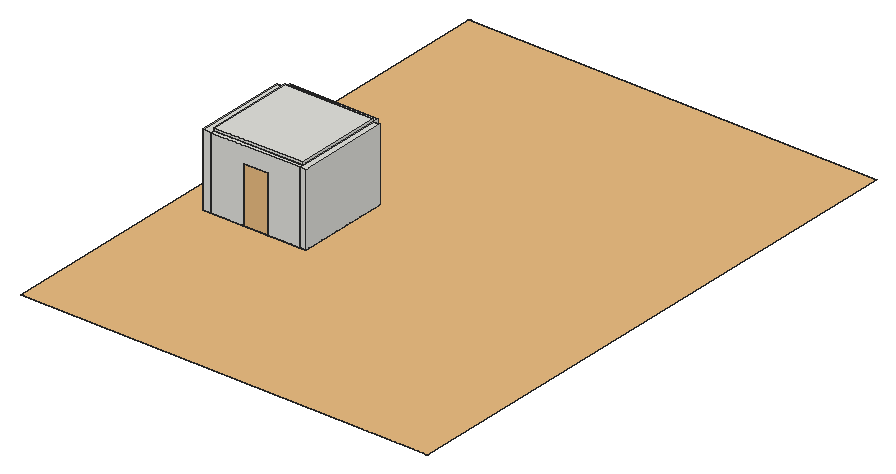
# SketchUp Ruby script. Lengths in inches.
U = 1.inch
M = Sketchup.active_model
def pt(a) = Geom::Point3d.new(a.map { |v| v * U })
def face(e, loops, mat)
  f = e.add_face(loops[0].map { |a| pt(a) })
  loops[1..].each { |l| e.add_face(l.map { |a| pt(a) }).erase! }
  f.material = f.back_material = mat if mat
  f
end
# faces: each face lists its corners as indices into pts; further lists are holes
def faces(e, pts, list, mat = nil) = list.each { |f| face(e, (f[0].is_a?(Array) ? f : [f]).map { |l| l.map { |i| pts[i] } }, mat) }
# xy, xz, yz: faces in a plane at the given z, y or x. An outline is a flat list of corners, or four numbers for a rectangle; further outlines are holes
def ring(l) = l.size == 4 ? [[l[0], l[1]], [l[2], l[1]], [l[2], l[3]], [l[0], l[3]]] : l.each_slice(2).to_a
def flat(e, list, mat, &to3) = list.each { |f| face(e, (f[0].is_a?(Array) ? f : [f]).map { |l| ring(l).map { |u, v| to3.(u, v) } }, mat) }
def xy(e, z, list, mat = nil) = flat(e, list, mat) { |x, y| [x, y, z] }
def xz(e, y, list, mat = nil) = flat(e, list, mat) { |x, z| [x, y, z] }
def yz(e, x, list, mat = nil) = flat(e, list, mat) { |y, z| [x, y, z] }
def lines(e, pts, list) = list.each { |a, b| e.add_line(pt(pts[a]), pt(pts[b])) }
# prism: a flat outline (further loops are holes) pulled along v
def prism(e, loops, v, mat = nil)
  f = face(e, loops, mat); d = Geom::Vector3d.new(v.map { |x| x * U })
  f.pushpull(f.normal.samedirection?(d) ? d.length : -d.length)
end
def box(e, o, s, mat = nil) = prism(e, [[o, [o[0] + s[0], o[1], o[2]], [o[0] + s[0], o[1] + s[1], o[2]], [o[0], o[1] + s[1], o[2]]]], [0, 0, s[2]], mat)
def at(x, y, z, deg = 0) = Geom::Transformation.translation(pt([x, y, z])) * Geom::Transformation.rotation(ORIGIN, Z_AXIS, deg.degrees)
def axes(o, x, y, z) = Geom::Transformation.new([*x, 0, *y, 0, *z, 0, *pt(o).to_a, 1])
def part(name) = M.definitions.add(name)
# library, detail: a bought-in or finely detailed component or shape, given as its bounding box
def library(name, o, s) = part(name).tap { |d| box(d.entities, o, s) }
def detail(e, o, s) = box(e.add_group.entities, o, s)
def put(e, d, t, mat = nil) = e.add_instance(d, t).tap { |i| i.material = mat if mat }
def group(e, t, mat = nil) = e.add_group.tap { |g| g.transformation = t; g.material = mat if mat }.entities
root = M.entities
M.materials.add("197_clay plaster pbr texture-seamless").color = [216, 205, 185]
M.materials.add("24_cement concrete tile texture-seamless").color = [228, 219, 211]
M.materials.add("30_cement concrete tile texture-seamless").color = [144, 72, 59]
M.materials.add("79_border traditional encaustic cement ornate tile texture-s").color = [183, 123, 111]
M.materials.add("Chrome_Black\#1").color = [42, 42, 42]
M.materials.add("Sumele_Skin").color = [140, 79, 58]
M.materials.add("[Color C08]").color = [102, 51, 0]
M.materials.add("[Color_003]").color = [170, 170, 170]
M.materials.add("seamless-bamboo-style-woven-pattern-with-a-natural-tradition").color = [200, 200, 200]
M.materials.add("verre blanc1").color = [248, 255, 255]
M.materials["verre blanc1"].alpha = 0.05
c1 = library("3d.dwg",[0,0,0],[608.51,837.33,0.01])
c2 = library("Basin with faucet",[0,-15.91,0],[23.7,18.47,14.64])
c3 = library("Pump bottle pair",[33.92,14.79,0],[6.24,3.49,7.05])
c4 = library("AROMATIZADOR ACQUAROMA",[-1.32,0,0],[3.68,2.36,8.56])
c5 = library("84714 Table Mirror Chic",[-3.54,-3.54,0],[7.08,7.08,13])
c6 = library("Vase with flowers",[-7.24,-6.22,5.67],[23.25,20.55,41.33])
c7 = library("Group\#12",[0,0,0],[22.57,47.9,32])
c8 = part("Vertical slat")
box(c8.entities,[0,0,0],[0.2,1,28.8])
c9 = part("Group\#13")
put(c9.entities,c8,at(0,12.75,0))
put(c9.entities,c8,at(0,1.27,0))
put(c9.entities,c8,at(0,10.2,0))
put(c9.entities,c8,at(0,8.92,0))
put(c9.entities,c8,at(0,6.375,0))
put(c9.entities,c8,at(0,11.47,0))
put(c9.entities,c8,at(0,5.1,0))
put(c9.entities,c8,at(0,2.55,0))
put(c9.entities,c8,at(0,7.65,0))
put(c9.entities,c8,at(0,3.82,0))
put(c9.entities,c8,at(0,0,0))
c10 = part("Vertical slat \#1")
box(c10.entities,[0,0,0],[1,0.2,28])
c11 = part("Group\#15")
put(c11.entities,c10,at(8.0625,0,0))
put(c11.entities,c10,at(9.41,0,0))
put(c11.entities,c10,at(4.03,0,0))
put(c11.entities,c10,at(10.75,0,0))
put(c11.entities,c10,at(1.34,0,0))
put(c11.entities,c10,at(2.6875,0,0))
put(c11.entities,c10,at(0,0,0))
put(c11.entities,c10,at(5.375,0,0))
put(c11.entities,c10,at(6.72,0,0))
c12 = library("Group\#62",[0,0,0],[1,23.9,36])
c13 = library("Group\#64",[0,0,0],[22.24,27.17,32.3125])
c14 = library("Group\#18",[-5.55,-2.43,0],[147.51,49.65,35.75])
c15 = part("Group\#22")
box(c15.entities,[0,0,0],[32.24,1,84])
c16 = library("Group\#43",[-54.65,-51.04,0],[147.99,489.25,189.39])
c17 = library("Group\#90",[0,0,0],[4,39.37,96])
put(root,c1,at(-40.22,-290.78,0))
put(root,c2,at(16.22,17.32,40,90))
put(root,c3,at(61.74,25.93,40,180),"Chrome_Black\#1")
put(root,c4,axes([16.42,10.53,40],[0,-1,0],[-1,0,0],[0,0,1]))
put(root,c5,axes([29.53,47.8,40],[-0.5,-0.86603,0],[-0.86603,0.5,0],[0,0,1]))
put(root,c6,axes([20.21,46.47,36.63],[-0.58344,-0.11447,0],[-0.11447,0.58344,0],[0,0,0.59456]))
g1 = group(root,at(0,0,0))
xy(g1,0,[[0,0,12,59.95],[0,59.95,12,137.9]])
xy(g1,108,[[0,0,12,137.9]])
xz(g1,0,[[0,0,12,108]])
xz(g1,137.9,[[0,0,12,108]])
yz(g1,0,[[0,0,137.9,108]])
yz(g1,12,[[0,0,137.9,4],[0,54,137.9,108]])
yz(g1,12,[[0,4,137.9,48]],"197_clay plaster pbr texture-seamless")
yz(g1,12,[[0,48,137.9,54]],"79_border traditional encaustic cement ornate tile texture-s")
g2 = group(root,at(12,137.9,0))
xy(g2,0,[[0,0,132,9.2]])
xy(g2,108,[[0,0,132,9.2]])
xz(g2,0,[[0,0,132,4],[0,54,132,108]])
xz(g2,0,[[0,4,132,48]],"197_clay plaster pbr texture-seamless")
xz(g2,0,[[0,48,132,54]],"79_border traditional encaustic cement ornate tile texture-s")
xz(g2,9.2,[[0,0,132,108]])
yz(g2,0,[[0,0,9.2,108]])
yz(g2,132,[[0,0,9.2,108]])
g3 = group(root,at(144,0,0))
xy(g3,0,[[0,0,9,137.9]])
xy(g3,108,[[0,0,9,137.9]])
xz(g3,0,[[0,0,9,108]])
xz(g3,137.9,[[0,0,9,108]])
yz(g3,0,[[0,0,137.9,4],[0,54,137.9,108]])
yz(g3,0,[[0,4,137.9,48]],"197_clay plaster pbr texture-seamless")
yz(g3,0,[[0,48,137.9,54]],"79_border traditional encaustic cement ornate tile texture-s")
yz(g3,9,[[0,0,137.9,108]])
g4 = group(root,at(12,0,0))
xy(g4,0,[[0,0,49.5,6],[85.5,0,132,6]])
xy(g4,84,[[49.5,0,85.5,6]])
xy(g4,108,[[0,0,132,6]])
xz(g4,0,[[0,0,49.5,0,49.5,84,85.5,84,85.5,0,132,0,132,108,0,108]])
xz(g4,6,[[0,0,49.5,4],[85.5,0,85.5,84,49.5,84,49.5,54,0,54,0,108,132,108,132,0]])
xz(g4,6,[[0,4,49.5,48]],"197_clay plaster pbr texture-seamless")
xz(g4,6,[[0,48,49.5,54]],"79_border traditional encaustic cement ornate tile texture-s")
yz(g4,0,[[0,0,6,108]])
yz(g4,49.5,[[0,0,6,84]])
yz(g4,85.5,[[0,0,6,84]])
yz(g4,132,[[0,0,6,108]])
g5 = group(root,at(0,0,-4),"24_cement concrete tile texture-seamless")
xy(g5,0,[[0,0,153,137.9]])
xy(g5,4,[[0,0,153,137.9]],"30_cement concrete tile texture-seamless")
xz(g5,0,[[0,0,153,4]])
xz(g5,137.9,[[0,0,153,4]])
yz(g5,0,[[0,0,137.9,4]])
yz(g5,153,[[0,0,137.9,4]])
put(root,c7,at(12,6,4),"Sumele_Skin")
g6 = group(root,at(128.8,20,0))
put(g6,c9,at(0,1.6,5.6),"Sumele_Skin")
put(g6,c9,at(0,18.55,5.6),"Sumele_Skin")
g7 = group(g6,at(0.2,0,0),"Sumele_Skin")
xy(g7,0,[[2,-14,15,33.9]])
xy(g7,4,[[2,-14,15,0],[0,0,2,16.95],[0,16.95,2,33.9]])
xy(g7,37,[[0,1,12,32.9]])
xy(g7,47,[[0,1,12,32.9]])
xy(g7,84,[[0,0,15,33.9]])
xz(g7,-14,[[2,0,15,4]])
xz(g7,0,[[0,4,15,84]])
xz(g7,1,[[0,37,12,47]])
xz(g7,32.9,[[0,37,12,47]])
xz(g7,33.9,[[2,0,2,4,0,4,0,84,15,84,15,0]])
yz(g7,0,[[[0.2,4.2,16.75,35.8],[1.6,5.6,15.35,34.4]],[[17.15,4.2,33.7,35.8],[18.55,5.6,32.3,34.4]],[1.6,5.6,15.35,34.4],[18.55,5.6,32.3,34.4],[[0.2,36.2,33.7,47.8],[1,37,32.9,47]],
  [[0.2,48.2,16.75,83.8],[3.6,49.6,13.35,49.6,13.61,49.62,13.87,49.67,14.12,49.75,14.35,49.87,14.57,50.01,14.76,50.1875,14.9375,50.38,15.08,50.6,15.2,50.83,15.28,51.08,15.33,51.34,15.35,51.6,15.35,80.4,15.33,80.66,15.28,80.92,15.2,81.17,15.08,81.4,14.9375,81.62,14.76,81.8125,14.57,81.99,14.35,82.13,14.12,82.25,13.87,82.33,13.61,82.38,13.35,82.4,3.6,82.4,3.34,82.38,3.08,82.33,2.83,82.25,2.6,82.13,2.38,81.99,2.1875,81.8125,2.01,81.62,1.87,81.4,1.75,81.17,1.67,80.92,1.62,80.66,1.6,80.4,1.6,51.6,1.62,51.34,1.67,51.08,1.75,50.83,1.87,50.6,2.01,50.38,2.1875,50.1875,2.38,50.01,2.6,49.87,2.83,49.75,3.08,49.67,3.34,49.62]],[[17.15,48.2,33.7,83.8],[20.55,49.6,30.3,49.6,30.5625,49.62,30.82,49.67,31.07,49.75,31.3,49.87,31.52,50.01,31.71,50.1875,31.89,50.38,32.03,50.6,32.15,50.83,32.23,51.08,32.28,51.34,32.3,51.6,32.3,80.4,32.28,80.66,32.23,80.92,32.15,81.17,32.03,81.4,31.89,81.62,31.71,81.8125,31.52,81.99,31.3,82.13,31.07,82.25,30.82,82.33,30.5625,82.38,30.3,82.4,20.55,82.4,20.29,82.38,20.03,82.33,19.78,82.25,19.55,82.13,19.33,81.99,19.14,81.8125,18.96,81.62,18.82,81.4,18.7,81.17,18.62,80.92,18.57,80.66,18.55,80.4,18.55,51.6,18.57,51.34,18.62,51.08,18.7,50.83,18.82,50.6,18.96,50.38,19.14,50.1875,19.33,50.01,19.55,49.87,19.78,49.75,20.03,49.67,20.29,49.62]]])
yz(g7,0,[[[0,4,16.95,36],[0.2,4.2,16.75,35.8]],[[16.95,4,33.9,36],[17.15,4.2,33.7,35.8]],[[0,36,33.9,48],[0.2,36.2,33.7,47.8]],[[0,48,16.95,84],[0.2,48.2,16.75,83.8]],[[16.95,48,33.9,84],[17.15,48.2,33.7,83.8]],
  [[3.6,49.6,3.34,49.62,3.08,49.67,2.83,49.75,2.6,49.87,2.38,50.01,2.1875,50.1875,2.01,50.38,1.87,50.6,1.75,50.83,1.67,51.08,1.62,51.34,1.6,51.6,1.6,80.4,1.62,80.66,1.67,80.92,1.75,81.17,1.87,81.4,2.01,81.62,2.1875,81.8125,2.38,81.99,2.6,82.13,2.83,82.25,3.08,82.33,3.34,82.38,3.6,82.4,13.35,82.4,13.61,82.38,13.87,82.33,14.12,82.25,14.35,82.13,14.57,81.99,14.76,81.8125,14.9375,81.62,15.08,81.4,15.2,81.17,15.28,80.92,15.33,80.66,15.35,80.4,15.35,51.6,15.33,51.34,15.28,51.08,15.2,50.83,15.08,50.6,14.9375,50.38,14.76,50.1875,14.57,50.01,14.35,49.87,14.12,49.75,13.87,49.67,13.61,49.62,13.35,49.6],[3.6,49.8,13.35,49.8,13.58,49.82,13.82,49.86,14.04,49.9375,14.25,50.04,14.45,50.17,14.62,50.33,14.78,50.5,14.91,50.7,15.01,50.91,15.09,51.13,15.13,51.37,15.15,51.6,15.15,80.4,15.13,80.63,15.09,80.87,15.01,81.09,14.91,81.3,14.78,81.5,14.62,81.67,14.45,81.83,14.25,81.96,14.04,82.0625,13.82,82.14,13.58,82.18,13.35,82.2,3.6,82.2,3.37,82.18,3.13,82.14,2.91,82.0625,2.7,81.96,2.5,81.83,2.33,81.67,2.17,81.5,2.04,81.3,1.9375,81.09,1.86,80.87,1.82,80.63,1.8,80.4,1.8,51.6,1.82,51.37,1.86,51.13,1.9375,50.91,2.04,50.7,2.17,50.5,2.33,50.33,2.5,50.17,2.7,50.04,2.91,49.9375,3.13,49.86,3.37,49.82]],[[20.55,49.6,20.29,49.62,20.03,49.67,19.78,49.75,19.55,49.87,19.33,50.01,19.14,50.1875,18.96,50.38,18.82,50.6,18.7,50.83,18.62,51.08,18.57,51.34,18.55,51.6,18.55,80.4,18.57,80.66,18.62,80.92,18.7,81.17,18.82,81.4,18.96,81.62,19.14,81.8125,19.33,81.99,19.55,82.13,19.78,82.25,20.03,82.33,20.29,82.38,20.55,82.4,30.3,82.4,30.5625,82.38,30.82,82.33,31.07,82.25,31.3,82.13,31.52,81.99,31.71,81.8125,31.89,81.62,32.03,81.4,32.15,81.17,32.23,80.92,32.28,80.66,32.3,80.4,32.3,51.6,32.28,51.34,32.23,51.08,32.15,50.83,32.03,50.6,31.89,50.38,31.71,50.1875,31.52,50.01,31.3,49.87,31.07,49.75,30.82,49.67,30.5625,49.62,30.3,49.6],[20.55,49.8,30.3,49.8,30.53,49.82,30.77,49.86,30.99,49.9375,31.2,50.04,31.4,50.17,31.57,50.33,31.73,50.5,31.86,50.7,31.96,50.91,32.04,51.13,32.08,51.37,32.1,51.6,32.1,80.4,32.08,80.63,32.04,80.87,31.96,81.09,31.86,81.3,31.73,81.5,31.57,81.67,31.4,81.83,31.2,81.96,30.99,82.0625,30.77,82.14,30.53,82.18,30.3,82.2,20.55,82.2,20.32,82.18,20.08,82.14,19.86,82.0625,19.65,81.96,19.45,81.83,19.28,81.67,19.12,81.5,18.99,81.3,18.89,81.09,18.8125,80.87,18.77,80.63,18.75,80.4,18.75,51.6,18.77,51.37,18.8125,51.13,18.89,50.91,18.99,50.7,19.12,50.5,19.28,50.33,19.45,50.17,19.65,50.04,19.86,49.9375,20.08,49.86,20.32,49.82]]],"[Color C08]")
yz(g7,0,[[3.6,49.8,3.37,49.82,3.13,49.86,2.91,49.9375,2.7,50.04,2.5,50.17,2.33,50.33,2.17,50.5,2.04,50.7,1.9375,50.91,1.86,51.13,1.82,51.37,1.8,51.6,1.8,80.4,1.82,80.63,1.86,80.87,1.9375,81.09,2.04,81.3,2.17,81.5,2.33,81.67,2.5,81.83,2.7,81.96,2.91,82.0625,3.13,82.14,3.37,82.18,3.6,82.2,13.35,82.2,13.58,82.18,13.82,82.14,14.04,82.0625,14.25,81.96,14.45,81.83,14.62,81.67,14.78,81.5,14.91,81.3,15.01,81.09,15.09,80.87,15.13,80.63,15.15,80.4,15.15,51.6,15.13,51.37,15.09,51.13,15.01,50.91,14.91,50.7,14.78,50.5,14.62,50.33,14.45,50.17,14.25,50.04,14.04,49.9375,13.82,49.86,13.58,49.82,13.35,49.8],[20.55,49.8,20.32,49.82,20.08,49.86,19.86,49.9375,19.65,50.04,19.45,50.17,19.28,50.33,19.12,50.5,18.99,50.7,18.89,50.91,18.8125,51.13,18.77,51.37,18.75,51.6,18.75,80.4,18.77,80.63,18.8125,80.87,18.89,81.09,18.99,81.3,19.12,81.5,19.28,81.67,19.45,81.83,19.65,81.96,19.86,82.0625,20.08,82.14,20.32,82.18,20.55,82.2,30.3,82.2,30.53,82.18,30.77,82.14,30.99,82.0625,31.2,81.96,31.4,81.83,31.57,81.67,31.73,81.5,31.86,81.3,31.96,81.09,32.04,80.87,32.08,80.63,32.1,80.4,32.1,51.6,32.08,51.37,32.04,51.13,31.96,50.91,31.86,50.7,31.73,50.5,31.57,50.33,31.4,50.17,31.2,50.04,30.99,49.9375,30.77,49.86,30.53,49.82,30.3,49.8]],"seamless-bamboo-style-woven-pattern-with-a-natural-tradition")
yz(g7,2,[[-14,0,33.9,4]])
yz(g7,12,[[1,37,32.9,47]])
yz(g7,15,[[-14,0,33.9,0,33.9,84,0,84,0,4,-14,4]])
g8 = group(root,at(97.5,6,0),"Sumele_Skin")
put(g8,c11,at(17.55,14,6.2))
put(g8,c11,at(2,14,6))
g9 = group(g8,at(0,0,0))
xy(g9,0,[[0,0,33.5,12]])
xy(g9,4,[[31.5,0,33.5,12],[0,12,15.75,14],[15.75,12,31.5,14]])
xy(g9,37.2,[[1.2,2,15.75,14],[15.75,2,30.3,14]],"Sumele_Skin")
xy(g9,46.8,[[1.2,2,15.75,14],[15.75,2,30.3,14]])
xy(g9,84,[[0,0,31.5,14]])
xz(g9,0,[[0,0,33.5,0,33.5,4,31.5,4,31.5,84,0,84]])
xz(g9,2,[[1.2,37.2,30.3,46.8]],"Sumele_Skin")
xz(g9,12,[[0,0,33.5,4]])
xz(g9,14,[[17.55,5.8,29.7,34.2],[2,6,13.75,34]])
xz(g9,14,[[[0.2,4.2,15.55,35.8],[2,6,13.75,34]],[[15.95,4.2,31.3,35.8],[17.55,5.8,29.7,34.2]],[[0.2,36.2,31.3,47.8],[1.2,37.2,30.3,46.8]],[[0.2,48.2,15.55,83.8],[4,50,11.75,50,12.01,50.02,12.27,50.07,12.52,50.15,12.75,50.27,12.97,50.41,13.16,50.59,13.34,50.78,13.48,51,13.6,51.23,13.68,51.48,13.73,51.74,13.75,52,13.75,80,13.73,80.26,13.68,80.52,13.6,80.77,13.48,81,13.34,81.22,13.16,81.41,12.97,81.59,12.75,81.73,12.52,81.85,12.27,81.93,12.01,81.98,11.75,82,4,82,3.74,81.98,3.48,81.93,3.23,81.85,3,81.73,2.78,81.59,2.59,81.41,2.41,81.22,2.27,81,2.15,80.77,2.07,80.52,2.02,80.26,2,80,2,52,2.02,51.74,2.07,51.48,2.15,51.23,2.27,51,2.41,50.78,2.59,50.59,2.78,50.41,3,50.27,3.23,50.15,3.48,50.07,3.74,50.02]],[[15.95,48.2,31.3,83.8],[19.75,50,27.5,50,27.76,50.02,28.02,50.07,28.27,50.15,28.5,50.27,28.72,50.41,28.91,50.59,29.09,50.78,29.23,51,29.35,51.23,29.43,51.48,29.48,51.74,29.5,52,29.5,80,29.48,80.26,29.43,80.52,29.35,80.77,29.23,81,29.09,81.22,28.91,81.41,28.72,81.59,28.5,81.73,28.27,81.85,28.02,81.93,27.76,81.98,27.5,82,19.75,82,19.49,81.98,19.23,81.93,18.98,81.85,18.75,81.73,18.53,81.59,18.34,81.41,18.16,81.22,18.02,81,17.9,80.77,17.82,80.52,17.77,80.26,17.75,80,17.75,52,17.77,51.74,17.82,51.48,17.9,51.23,18.02,51,18.16,50.78,18.34,50.59,18.53,50.41,18.75,50.27,18.98,50.15,19.23,50.07,19.49,50.02]]],"Sumele_Skin")
xz(g9,14,[[[0,4,15.75,36],[0.2,4.2,15.55,35.8]],[[15.75,4,31.5,36],[15.95,4.2,31.3,35.8]],[[0,36,31.5,48],[0.2,36.2,31.3,47.8]],[[0,48,15.75,84],[0.2,48.2,15.55,83.8]],[[15.75,48,31.5,84],[15.95,48.2,31.3,83.8]],
  [[4,50,3.74,50.02,3.48,50.07,3.23,50.15,3,50.27,2.78,50.41,2.59,50.59,2.41,50.78,2.27,51,2.15,51.23,2.07,51.48,2.02,51.74,2,52,2,80,2.02,80.26,2.07,80.52,2.15,80.77,2.27,81,2.41,81.22,2.59,81.41,2.78,81.59,3,81.73,3.23,81.85,3.48,81.93,3.74,81.98,4,82,11.75,82,12.01,81.98,12.27,81.93,12.52,81.85,12.75,81.73,12.97,81.59,13.16,81.41,13.34,81.22,13.48,81,13.6,80.77,13.68,80.52,13.73,80.26,13.75,80,13.75,52,13.73,51.74,13.68,51.48,13.6,51.23,13.48,51,13.34,50.78,13.16,50.59,12.97,50.41,12.75,50.27,12.52,50.15,12.27,50.07,12.01,50.02,11.75,50],[4,50.2,11.75,50.2,11.98,50.22,12.22,50.26,12.4375,50.34,12.65,50.44,12.85,50.57,13.02,50.73,13.18,50.9,13.31,51.1,13.41,51.3125,13.49,51.53,13.53,51.77,13.55,52,13.55,80,13.53,80.23,13.49,80.47,13.41,80.6875,13.31,80.9,13.18,81.1,13.02,81.27,12.85,81.43,12.65,81.56,12.4375,81.66,12.22,81.74,11.98,81.78,11.75,81.8,4,81.8,3.77,81.78,3.53,81.74,3.3125,81.66,3.1,81.56,2.9,81.43,2.73,81.27,2.57,81.1,2.44,80.9,2.34,80.6875,2.26,80.47,2.22,80.23,2.2,80,2.2,52,2.22,51.77,2.26,51.53,2.34,51.3125,2.44,51.1,2.57,50.9,2.73,50.73,2.9,50.57,3.1,50.44,3.3125,50.34,3.53,50.26,3.77,50.22]],[[19.75,50,19.49,50.02,19.23,50.07,18.98,50.15,18.75,50.27,18.53,50.41,18.34,50.59,18.16,50.78,18.02,51,17.9,51.23,17.82,51.48,17.77,51.74,17.75,52,17.75,80,17.77,80.26,17.82,80.52,17.9,80.77,18.02,81,18.16,81.22,18.34,81.41,18.53,81.59,18.75,81.73,18.98,81.85,19.23,81.93,19.49,81.98,19.75,82,27.5,82,27.76,81.98,28.02,81.93,28.27,81.85,28.5,81.73,28.72,81.59,28.91,81.41,29.09,81.22,29.23,81,29.35,80.77,29.43,80.52,29.48,80.26,29.5,80,29.5,52,29.48,51.74,29.43,51.48,29.35,51.23,29.23,51,29.09,50.78,28.91,50.59,28.72,50.41,28.5,50.27,28.27,50.15,28.02,50.07,27.76,50.02,27.5,50],[19.75,50.2,27.5,50.2,27.73,50.22,27.97,50.26,28.1875,50.34,28.4,50.44,28.6,50.57,28.77,50.73,28.93,50.9,29.06,51.1,29.16,51.3125,29.24,51.53,29.28,51.77,29.3,52,29.3,80,29.28,80.23,29.24,80.47,29.16,80.6875,29.06,80.9,28.93,81.1,28.77,81.27,28.6,81.43,28.4,81.56,28.1875,81.66,27.97,81.74,27.73,81.78,27.5,81.8,19.75,81.8,19.52,81.78,19.28,81.74,19.0625,81.66,18.85,81.56,18.65,81.43,18.48,81.27,18.32,81.1,18.19,80.9,18.09,80.6875,18.01,80.47,17.97,80.23,17.95,80,17.95,52,17.97,51.77,18.01,51.53,18.09,51.3125,18.19,51.1,18.32,50.9,18.48,50.73,18.65,50.57,18.85,50.44,19.0625,50.34,19.28,50.26,19.52,50.22]]],"[Color C08]")
xz(g9,14,[[4,50.2,3.77,50.22,3.53,50.26,3.3125,50.34,3.1,50.44,2.9,50.57,2.73,50.73,2.57,50.9,2.44,51.1,2.34,51.3125,2.26,51.53,2.22,51.77,2.2,52,2.2,80,2.22,80.23,2.26,80.47,2.34,80.6875,2.44,80.9,2.57,81.1,2.73,81.27,2.9,81.43,3.1,81.56,3.3125,81.66,3.53,81.74,3.77,81.78,4,81.8,11.75,81.8,11.98,81.78,12.22,81.74,12.4375,81.66,12.65,81.56,12.85,81.43,13.02,81.27,13.18,81.1,13.31,80.9,13.41,80.6875,13.49,80.47,13.53,80.23,13.55,80,13.55,52,13.53,51.77,13.49,51.53,13.41,51.3125,13.31,51.1,13.18,50.9,13.02,50.73,12.85,50.57,12.65,50.44,12.4375,50.34,12.22,50.26,11.98,50.22,11.75,50.2],[19.75,50.2,19.52,50.22,19.28,50.26,19.0625,50.34,18.85,50.44,18.65,50.57,18.48,50.73,18.32,50.9,18.19,51.1,18.09,51.3125,18.01,51.53,17.97,51.77,17.95,52,17.95,80,17.97,80.23,18.01,80.47,18.09,80.6875,18.19,80.9,18.32,81.1,18.48,81.27,18.65,81.43,18.85,81.56,19.0625,81.66,19.28,81.74,19.52,81.78,19.75,81.8,27.5,81.8,27.73,81.78,27.97,81.74,28.1875,81.66,28.4,81.56,28.6,81.43,28.77,81.27,28.93,81.1,29.06,80.9,29.16,80.6875,29.24,80.47,29.28,80.23,29.3,80,29.3,52,29.28,51.77,29.24,51.53,29.16,51.3125,29.06,51.1,28.93,50.9,28.77,50.73,28.6,50.57,28.4,50.44,28.1875,50.34,27.97,50.26,27.73,50.22,27.5,50.2]],"seamless-bamboo-style-woven-pattern-with-a-natural-tradition")
yz(g9,0,[[0,0,0,84,14,84,14,4,12,4,12,0]],"Sumele_Skin")
yz(g9,1.2,[[2,37.2,14,46.8]])
yz(g9,30.3,[[2,37.2,14,46.8]],"Sumele_Skin")
yz(g9,31.5,[[0,4,14,84]])
yz(g9,33.5,[[0,0,12,4]])
g10 = group(root,at(12,6,36))
box(g10,[0,0,0],[22.375,47.9,4])
put(root,c12,at(12,16.28,51.25))
put(root,c13,at(10.77,66.78,0))
put(root,c14,at(145.45,135.47,0,-180))
put(root,c15,at(12,94.9,0),"verre blanc1")
g11 = group(root,at(12,53.9,0))
prism(g11,[[[0,0,0],[32.22,0,0],[32.22,0,84],[0,0,84]],[[30.62,0,1.6],[1.6,0,1.6],[1.6,0,82.4],[30.62,0,82.4]]],[0,1,0])
g12 = group(root,at(13.6,53.9,1.6),"Sumele_Skin")
box(g12,[0,0,0],[29.02,1,38.4])
g13 = group(root,at(13.6,54.1,40),"verre blanc1")
box(g13,[0,0,0],[29.02,0.6,42.4])
put(root,c15,at(111.78,94.9,0),"verre blanc1")
put(root,c15,at(111.78,53.9,0),"verre blanc1")
put(root,c16,axes([125.0625,72.07,40.18],[0,0.1,0],[0,0,0.1],[0.1,0,0]),"[Color_003]")
g14 = group(root,at(12,6,108))
box(g14,[0,0,0],[132,131.9,4])
put(root,c17,axes([61.5,0,0],[0,1,0],[0.9144,0,0],[0,0,0.875]))
